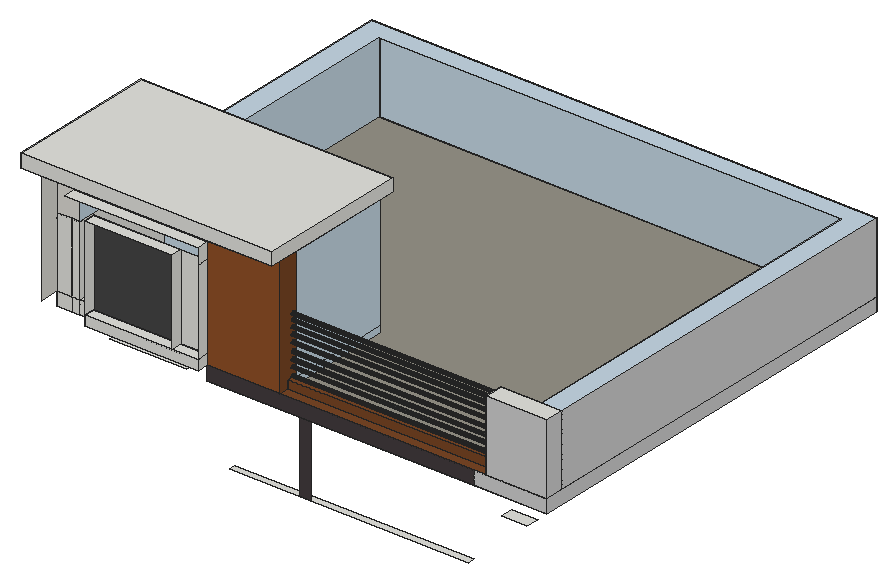
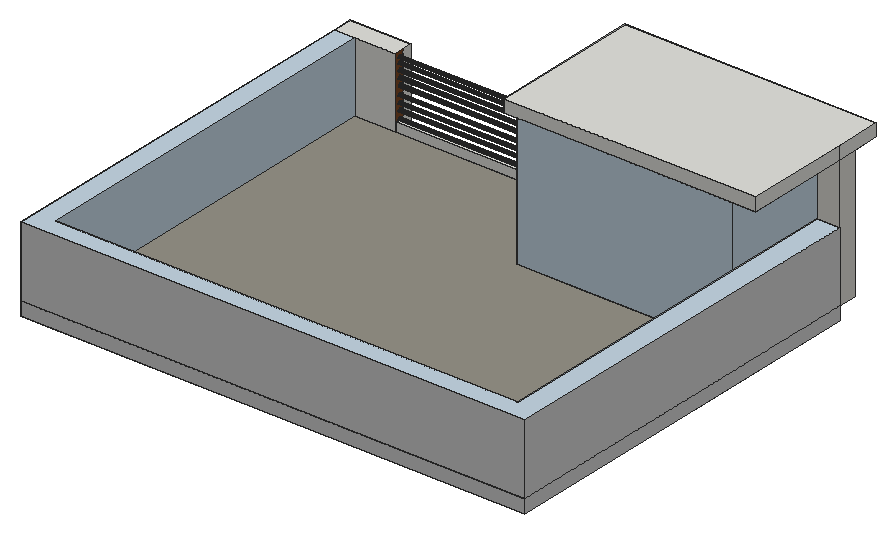
# SketchUp Ruby script. Lengths in inches.
U = 1.inch
M = Sketchup.active_model
def pt(a) = Geom::Point3d.new(a.map { |v| v * U })
def face(e, loops, mat)
  f = e.add_face(loops[0].map { |a| pt(a) })
  loops[1..].each { |l| e.add_face(l.map { |a| pt(a) }).erase! }
  f.material = f.back_material = mat if mat
  f
end
# faces: each face lists its corners as indices into pts; further lists are holes
def faces(e, pts, list, mat = nil) = list.each { |f| face(e, (f[0].is_a?(Array) ? f : [f]).map { |l| l.map { |i| pts[i] } }, mat) }
# xy, xz, yz: faces in a plane at the given z, y or x. An outline is a flat list of corners, or four numbers for a rectangle; further outlines are holes
def ring(l) = l.size == 4 ? [[l[0], l[1]], [l[2], l[1]], [l[2], l[3]], [l[0], l[3]]] : l.each_slice(2).to_a
def flat(e, list, mat, &to3) = list.each { |f| face(e, (f[0].is_a?(Array) ? f : [f]).map { |l| ring(l).map { |u, v| to3.(u, v) } }, mat) }
def xy(e, z, list, mat = nil) = flat(e, list, mat) { |x, y| [x, y, z] }
def xz(e, y, list, mat = nil) = flat(e, list, mat) { |x, z| [x, y, z] }
def yz(e, x, list, mat = nil) = flat(e, list, mat) { |y, z| [x, y, z] }
def lines(e, pts, list) = list.each { |a, b| e.add_line(pt(pts[a]), pt(pts[b])) }
# prism: a flat outline (further loops are holes) pulled along v
def prism(e, loops, v, mat = nil)
  f = face(e, loops, mat); d = Geom::Vector3d.new(v.map { |x| x * U })
  f.pushpull(f.normal.samedirection?(d) ? d.length : -d.length)
end
def box(e, o, s, mat = nil) = prism(e, [[o, [o[0] + s[0], o[1], o[2]], [o[0] + s[0], o[1] + s[1], o[2]], [o[0], o[1] + s[1], o[2]]]], [0, 0, s[2]], mat)
def at(x, y, z, deg = 0) = Geom::Transformation.translation(pt([x, y, z])) * Geom::Transformation.rotation(ORIGIN, Z_AXIS, deg.degrees)
def axes(o, x, y, z) = Geom::Transformation.new([*x, 0, *y, 0, *z, 0, *pt(o).to_a, 1])
def part(name) = M.definitions.add(name)
# library, detail: a bought-in or finely detailed component or shape, given as its bounding box
def library(name, o, s) = part(name).tap { |d| box(d.entities, o, s) }
def detail(e, o, s) = box(e.add_group.entities, o, s)
def put(e, d, t, mat = nil) = e.add_instance(d, t).tap { |i| i.material = mat if mat }
def group(e, t, mat = nil) = e.add_group.tap { |g| g.transformation = t; g.material = mat if mat }.entities
root = M.entities
M.materials.add("[Asphalt New]").color = [67, 60, 62]
M.materials.add("[Carrera Marble]").color = [207, 207, 207]
M.materials.add("[Color M07]").color = [58, 58, 58]
M.materials.add("[Formica Graystone]").color = [149, 146, 135]
M.materials.add("[Formica Laminate Dark]").color = [50, 53, 60]
M.materials.add("[Formica Laminate Light]").color = [213, 189, 164]
M.materials.add("[Granite Dark Gray]").color = [69, 68, 68]
M.materials.add("[Mirror 02]").color = [229, 229, 229]
M.materials.add("[Terrazzo Light Blue]").color = [196, 214, 227]
M.materials.add("[Terrazzo Tile Light]").color = [219, 217, 210]
M.materials.add("[Translucent Glass Gray]").color = [96, 96, 96]
M.materials["[Translucent Glass Gray]"].alpha = 0.5
M.materials.add("[Wood Cherry Original]").color = [142, 80, 39]
M.materials.add("[Wood Veneer 01]").color = [120, 70, 37]
xy(root,337.375,[[155.47,113.77,364.18,119.67]])
xy(root,386.13,[[143.73,278.02,202.85,283.21]])
xy(root,387.97,[[397.72,107.86,419.72,119.36]])
xy(root,407.4375,[[144.47,102.9,155.47,119.67],[421.41,102.9,440.93,107.86],[376,107.86,421.41,119.67],[421.41,107.86,440.93,119.67],[0,119.67,19.52,278.02],
  [421.41,119.67,440.93,278.02],[0,278.02,19.52,291.29],[19.52,278.02,378.85,291.29],[378.85,278.02,421.41,291.29],[421.41,278.02,440.93,291.29],
  [0,291.29,19.52,462.9],[19.52,291.29,365.25,443.38],[365.25,291.29,378.85,443.38],[378.85,291.29,421.41,443.38],[421.41,291.29,440.93,462.9],
  [19.52,443.38,365.25,462.9],[365.25,443.38,378.85,462.9],[378.85,443.38,421.41,462.9]])
xy(root,407.4375,[[[155.47,102.9,155.47,119.67,19.52,119.67,19.52,278.02,421.41,278.02,421.41,119.67,364.18,119.67,364.18,107.86,421.41,107.86,421.41,102.9],[216.29,107.86,226.02,113.77]]],"[Formica Laminate Light]")
xy(root,409.91,[[59.64,102.9,126.33,116.97]])
xy(root,419.375,[[45.1,93.15,144.47,102.9],[387.7,102.9,440.93,119.67],[207.97,111.29,387.7,119.67],[0,119.67,0,462.9,440.93,462.9,440.93,119.67,423.04,119.67,423.04,446.61,19.52,446.61,19.52,119.67],[19.52,119.67,144.47,211.42],
  [144.47,119.67,207.97,211.42]])
xy(root,419.375,[[207.97,119.67,423.04,119.67,423.04,446.61,19.52,446.61,19.52,211.42,207.97,211.42]],"[Formica Graystone]")
xy(root,419.375,[[207.97,102.9,387.7,111.29]],"[Wood Veneer 01]")
xy(root,426.94,[[207.97,116.04,387.7,119.67]])
xy(root,426.94,[[207.97,111.29,387.7,116.04]],"[Wood Veneer 01]")
xy(root,428.03,[[45.1,93.15,121.39,102.9],[121.39,93.15,144.47,102.9]])
xy(root,480.75,[[387.7,102.9,440.93,119.67]])
xy(root,480.75,[[0,119.67,19.52,119.67,19.52,446.61,423.04,446.61,423.04,119.67,440.93,119.67,440.93,462.9,0,462.9]],"[Terrazzo Light Blue]")
xy(root,501.96,[[45.1,93.15,121.39,102.9]])
xy(root,515.65,[[27.95,93.15,144.47,102.9]])
xy(root,533.5625,[[0,79.34,144.47,102.9],[144.47,79.34,207.97,102.9],[207.97,79.34,219.41,119.67],[0,102.9,0,119.67,19.52,119.67,19.52,211.42,207.97,211.42,207.97,102.9],[0,119.67,19.52,211.42],
  [207.97,119.67,219.41,211.42]])
xy(root,544.875,[[0,79.34,219.41,211.42]])
xz(root,79.34,[[0,533.5625,219.41,544.875]])
xz(root,93.15,[[45.1,419.375,144.47,428.03]])
xz(root,102.9,[[45.1,419.375,144.47,428.03],[121.39,428.03,144.47,501.96]])
xz(root,102.9,[[144.47,407.4375,377.08,419.375]],"[Asphalt New]")
xz(root,102.9,[[377.08,407.4375,440.93,419.375],[387.7,419.375,440.93,480.75]],"[Carrera Marble]")
xz(root,102.9,[[45.1,428.03,121.39,501.96]],"[Granite Dark Gray]")
xz(root,102.9,[[144.47,419.375,207.97,533.5625]],"[Wood Cherry Original]")
xz(root,111.29,[[207.97,419.375,387.7,426.94]],"[Wood Veneer 01]")
xz(root,113.77,[[216.29,337.375,226.02,407.4375]],"[Asphalt New]")
xz(root,119.67,[[0,407.4375,12.41,419.375],[12.41,407.4375,12.51,419.375],[12.51,407.4375,19.52,419.375],[19.52,407.4375,144.47,419.375],[0,419.375,12.41,480.75],
  [12.41,419.375,12.51,480.75],[12.51,419.375,19.52,480.75],[207.97,419.375,387.7,426.94],[387.7,419.375,423.04,480.75],[423.04,419.375,440.93,480.75]])
xz(root,119.67,[[0,480.75,19.52,533.5625]],"[Terrazzo Tile Light]")
xz(root,211.42,[[0,533.5625,219.41,544.875]])
xz(root,211.42,[[19.52,419.375,207.97,533.5625]],"[Terrazzo Light Blue]")
xz(root,278.02,[[263.57,345.67,290.95,362.74],[292.74,345.67,324.88,362.74],[263.57,365.24,290.95,384.78],[292.74,365.24,324.88,384.78]],"[Mirror 02]")
xz(root,283.21,[[170.75,329.99,173.63,383.16]],"[Formica Laminate Dark]")
xz(root,283.21,[[146.7,329.99,170.75,383.16],[173.63,329.99,199.875,383.16]],"[Translucent Glass Gray]")
xz(root,446.61,[[19.52,419.375,20.91,480.75]])
xz(root,446.61,[[20.91,419.375,423.04,480.75]],"[Terrazzo Light Blue]")
xz(root,462.9,[[0,407.4375,440.93,419.375],[0,419.375,440.93,480.75]],"[Carrera Marble]")
yz(root,0,[[79.34,533.5625,119.67,544.875],[119.67,533.5625,211.42,544.875]])
yz(root,0,[[119.67,407.4375,462.9,419.375],[119.67,419.375,462.9,480.75]],"[Carrera Marble]")
yz(root,0,[[102.9,419.375,119.67,533.5625]],"[Terrazzo Tile Light]")
yz(root,19.52,[[119.67,419.375,211.42,480.75]])
yz(root,19.52,[[211.42,419.375,446.61,480.75],[119.67,480.75,211.42,533.5625]],"[Terrazzo Light Blue]")
yz(root,45.1,[[93.15,419.375,102.9,428.03],[93.15,428.03,102.9,501.96]])
yz(root,121.39,[[93.15,428.03,102.9,501.96]])
yz(root,144.47,[[93.15,419.375,102.9,428.03],[93.15,428.03,102.9,501.96],[93.15,501.96,102.9,515.65]])
yz(root,207.97,[[111.29,419.375,119.67,426.94]])
yz(root,207.97,[[119.67,419.375,211.42,425],[119.67,425,211.42,533.5625]],"[Terrazzo Light Blue]")
yz(root,207.97,[[[102.9,419.375,111.29,419.375,111.29,426.94,119.67,426.94,119.67,533.5625,102.9,533.5625],[116.04,475.69,115.71,475.73,115.41,475.85,115.15,476.05,114.96,476.31,114.83,476.61,114.79,476.94,114.83,477.26,114.96,477.56,115.15,477.82,115.41,478.02,115.71,478.14,116.04,478.19,116.36,478.14,116.66,478.02,116.92,477.82,117.12,477.56,117.25,477.26,117.29,476.94,117.25,476.61,117.12,476.31,116.92,476.05,116.66,475.85,116.36,475.73],[116.04,470.81,115.71,470.85,115.41,470.98,115.15,471.18,114.96,471.44,114.83,471.74,114.79,472.06,114.83,472.38,114.96,472.69,115.15,472.94,115.41,473.14,115.71,473.27,116.04,473.31,116.36,473.27,116.66,473.14,116.92,472.94,117.12,472.69,117.25,472.38,117.29,472.06,117.25,471.74,117.12,471.44,116.92,471.18,116.66,470.98,116.36,470.85],[116.04,465.19,115.71,465.23,115.41,465.35,115.15,465.55,114.96,465.81,114.83,466.11,114.79,466.44,114.83,466.76,114.96,467.06,115.15,467.32,115.41,467.52,115.71,467.64,116.04,467.69,116.36,467.64,116.66,467.52,116.92,467.32,117.12,467.06,117.25,466.76,117.29,466.44,117.25,466.11,117.12,465.81,116.92,465.55,116.66,465.35,116.36,465.23],[116.04,459.44,115.71,459.48,115.41,459.6,115.15,459.8,114.96,460.06,114.83,460.36,114.79,460.69,114.83,461.01,114.96,461.31,115.15,461.57,115.41,461.77,115.71,461.89,116.04,461.94,116.36,461.89,116.66,461.77,116.92,461.57,117.12,461.31,117.25,461.01,117.29,460.69,117.25,460.36,117.12,460.06,116.92,459.8,116.66,459.6,116.36,459.48],[116.04,453.19,115.71,453.23,115.41,453.35,115.15,453.55,114.96,453.81,114.83,454.11,114.79,454.44,114.83,454.76,114.96,455.06,115.15,455.32,115.41,455.52,115.71,455.64,116.04,455.69,116.36,455.64,116.66,455.52,116.92,455.32,117.12,455.06,117.25,454.76,117.29,454.44,117.25,454.11,117.12,453.81,116.92,453.55,116.66,453.35,116.36,453.23],[116.04,446,115.71,446.04,115.41,446.17,115.15,446.36,114.96,446.62,114.83,446.92,114.79,447.25,114.83,447.57,114.96,447.87,115.15,448.13,115.41,448.33,115.71,448.45,116.04,448.5,116.36,448.45,116.66,448.33,116.92,448.13,117.12,447.87,117.25,447.57,117.29,447.25,117.25,446.92,117.12,446.62,116.92,446.36,116.66,446.17,116.36,446.04],[116.04,426.94,115.71,426.98,115.41,427.1,115.15,427.3,114.96,427.56,114.83,427.86,114.79,428.19,114.83,428.51,114.96,428.81,115.15,429.07,115.41,429.27,115.71,429.39,116.04,429.44,116.36,429.39,116.66,429.27,116.92,429.07,117.12,428.81,117.25,428.51,117.29,428.19,117.25,427.86,117.12,427.56,116.92,427.3,116.66,427.1,116.36,426.98],[116.04,433.87,115.71,433.92,115.41,434.04,115.15,434.24,114.96,434.5,114.83,434.8,114.79,435.12,114.83,435.45,114.96,435.75,115.15,436.01,115.41,436.21,115.71,436.33,116.04,436.37,116.36,436.33,116.66,436.21,116.92,436.01,117.12,435.75,117.25,435.45,117.29,435.12,117.25,434.8,117.12,434.5,116.92,434.24,116.66,434.04,116.36,433.92],[116.04,439.69,115.71,439.73,115.41,439.85,115.15,440.05,114.96,440.31,114.83,440.61,114.79,440.94,114.83,441.26,114.96,441.56,115.15,441.82,115.41,442.02,115.71,442.14,116.04,442.19,116.36,442.14,116.66,442.02,116.92,441.82,117.12,441.56,117.25,441.26,117.29,440.94,117.25,440.61,117.12,440.31,116.92,440.05,116.66,439.85,116.36,439.73]]],"[Wood Veneer 01]")
yz(root,219.41,[[79.34,533.5625,211.42,544.875]])
yz(root,387.7,[[102.9,419.375,111.29,480.75],[111.29,419.375,119.67,426.94],[116.04,426.94,116.36,426.98,116.66,427.1,116.92,427.3,117.12,427.56,117.25,427.86,117.29,428.19,117.25,428.51,117.12,428.81,116.92,429.07,116.66,429.27,116.36,429.39,116.04,429.44,115.71,429.39,115.41,429.27,115.15,429.07,114.96,428.81,114.83,428.51,114.79,428.19,114.83,427.86,114.96,427.56,115.15,427.3,115.41,427.1,115.71,426.98],[116.04,433.87,116.36,433.92,116.66,434.04,116.92,434.24,117.12,434.5,117.25,434.8,117.29,435.12,117.25,435.45,117.12,435.75,116.92,436.01,116.66,436.21,116.36,436.33,116.04,436.37,115.71,436.33,115.41,436.21,115.15,436.01,114.96,435.75,114.83,435.45,114.79,435.12,114.83,434.8,114.96,434.5,115.15,434.24,115.41,434.04,115.71,433.92],[116.04,439.69,116.36,439.73,116.66,439.85,116.92,440.05,117.12,440.31,117.25,440.61,117.29,440.94,117.25,441.26,117.12,441.56,116.92,441.82,116.66,442.02,116.36,442.14,116.04,442.19,115.71,442.14,115.41,442.02,115.15,441.82,114.96,441.56,114.83,441.26,114.79,440.94,114.83,440.61,114.96,440.31,115.15,440.05,115.41,439.85,115.71,439.73],
  [116.04,446,116.36,446.04,116.66,446.17,116.92,446.36,117.12,446.62,117.25,446.92,117.29,447.25,117.25,447.57,117.12,447.87,116.92,448.13,116.66,448.33,116.36,448.45,116.04,448.5,115.71,448.45,115.41,448.33,115.15,448.13,114.96,447.87,114.83,447.57,114.79,447.25,114.83,446.92,114.96,446.62,115.15,446.36,115.41,446.17,115.71,446.04],[116.04,453.19,116.36,453.23,116.66,453.35,116.92,453.55,117.12,453.81,117.25,454.11,117.29,454.44,117.25,454.76,117.12,455.06,116.92,455.32,116.66,455.52,116.36,455.64,116.04,455.69,115.71,455.64,115.41,455.52,115.15,455.32,114.96,455.06,114.83,454.76,114.79,454.44,114.83,454.11,114.96,453.81,115.15,453.55,115.41,453.35,115.71,453.23],[116.04,459.44,116.36,459.48,116.66,459.6,116.92,459.8,117.12,460.06,117.25,460.36,117.29,460.69,117.25,461.01,117.12,461.31,116.92,461.57,116.66,461.77,116.36,461.89,116.04,461.94,115.71,461.89,115.41,461.77,115.15,461.57,114.96,461.31,114.83,461.01,114.79,460.69,114.83,460.36,114.96,460.06,115.15,459.8,115.41,459.6,115.71,459.48],[116.04,465.19,116.36,465.23,116.66,465.35,116.92,465.55,117.12,465.81,117.25,466.11,117.29,466.44,117.25,466.76,117.12,467.06,116.92,467.32,116.66,467.52,116.36,467.64,116.04,467.69,115.71,467.64,115.41,467.52,115.15,467.32,114.96,467.06,114.83,466.76,114.79,466.44,114.83,466.11,114.96,465.81,115.15,465.55,115.41,465.35,115.71,465.23],[116.04,470.81,116.36,470.85,116.66,470.98,116.92,471.18,117.12,471.44,117.25,471.74,117.29,472.06,117.25,472.38,117.12,472.69,116.92,472.94,116.66,473.14,116.36,473.27,116.04,473.31,115.71,473.27,115.41,473.14,115.15,472.94,114.96,472.69,114.83,472.38,114.79,472.06,114.83,471.74,114.96,471.44,115.15,471.18,115.41,470.98,115.71,470.85],
  [116.04,475.69,116.36,475.73,116.66,475.85,116.92,476.05,117.12,476.31,117.25,476.61,117.29,476.94,117.25,477.26,117.12,477.56,116.92,477.82,116.66,478.02,116.36,478.14,116.04,478.19,115.71,478.14,115.41,478.02,115.15,477.82,114.96,477.56,114.83,477.26,114.79,476.94,114.83,476.61,114.96,476.31,115.15,476.05,115.41,475.85,115.71,475.73]])
yz(root,387.7,[[[111.29,426.94,119.67,480.75],[116.04,475.69,116.36,475.73,116.66,475.85,116.92,476.05,117.12,476.31,117.25,476.61,117.29,476.94,117.25,477.26,117.12,477.56,116.92,477.82,116.66,478.02,116.36,478.14,116.04,478.19,115.71,478.14,115.41,478.02,115.15,477.82,114.96,477.56,114.83,477.26,114.79,476.94,114.83,476.61,114.96,476.31,115.15,476.05,115.41,475.85,115.71,475.73],[116.04,426.94,116.36,426.98,116.66,427.1,116.92,427.3,117.12,427.56,117.25,427.86,117.29,428.19,117.25,428.51,117.12,428.81,116.92,429.07,116.66,429.27,116.36,429.39,116.04,429.44,115.71,429.39,115.41,429.27,115.15,429.07,114.96,428.81,114.83,428.51,114.79,428.19,114.83,427.86,114.96,427.56,115.15,427.3,115.41,427.1,115.71,426.98],[116.04,470.81,116.36,470.85,116.66,470.98,116.92,471.18,117.12,471.44,117.25,471.74,117.29,472.06,117.25,472.38,117.12,472.69,116.92,472.94,116.66,473.14,116.36,473.27,116.04,473.31,115.71,473.27,115.41,473.14,115.15,472.94,114.96,472.69,114.83,472.38,114.79,472.06,114.83,471.74,114.96,471.44,115.15,471.18,115.41,470.98,115.71,470.85],[116.04,433.87,116.36,433.92,116.66,434.04,116.92,434.24,117.12,434.5,117.25,434.8,117.29,435.12,117.25,435.45,117.12,435.75,116.92,436.01,116.66,436.21,116.36,436.33,116.04,436.37,115.71,436.33,115.41,436.21,115.15,436.01,114.96,435.75,114.83,435.45,114.79,435.12,114.83,434.8,114.96,434.5,115.15,434.24,115.41,434.04,115.71,433.92],[116.04,465.19,116.36,465.23,116.66,465.35,116.92,465.55,117.12,465.81,117.25,466.11,117.29,466.44,117.25,466.76,117.12,467.06,116.92,467.32,116.66,467.52,116.36,467.64,116.04,467.69,115.71,467.64,115.41,467.52,115.15,467.32,114.96,467.06,114.83,466.76,114.79,466.44,114.83,466.11,114.96,465.81,115.15,465.55,115.41,465.35,115.71,465.23],[116.04,439.69,116.36,439.73,116.66,439.85,116.92,440.05,117.12,440.31,117.25,440.61,117.29,440.94,117.25,441.26,117.12,441.56,116.92,441.82,116.66,442.02,116.36,442.14,116.04,442.19,115.71,442.14,115.41,442.02,115.15,441.82,114.96,441.56,114.83,441.26,114.79,440.94,114.83,440.61,114.96,440.31,115.15,440.05,115.41,439.85,115.71,439.73],[116.04,459.44,116.36,459.48,116.66,459.6,116.92,459.8,117.12,460.06,117.25,460.36,117.29,460.69,117.25,461.01,117.12,461.31,116.92,461.57,116.66,461.77,116.36,461.89,116.04,461.94,115.71,461.89,115.41,461.77,115.15,461.57,114.96,461.31,114.83,461.01,114.79,460.69,114.83,460.36,114.96,460.06,115.15,459.8,115.41,459.6,115.71,459.48],[116.04,446,116.36,446.04,116.66,446.17,116.92,446.36,117.12,446.62,117.25,446.92,117.29,447.25,117.25,447.57,117.12,447.87,116.92,448.13,116.66,448.33,116.36,448.45,116.04,448.5,115.71,448.45,115.41,448.33,115.15,448.13,114.96,447.87,114.83,447.57,114.79,447.25,114.83,446.92,114.96,446.62,115.15,446.36,115.41,446.17,115.71,446.04],[116.04,453.19,116.36,453.23,116.66,453.35,116.92,453.55,117.12,453.81,117.25,454.11,117.29,454.44,117.25,454.76,117.12,455.06,116.92,455.32,116.66,455.52,116.36,455.64,116.04,455.69,115.71,455.64,115.41,455.52,115.15,455.32,114.96,455.06,114.83,454.76,114.79,454.44,114.83,454.11,114.96,453.81,115.15,453.55,115.41,453.35,115.71,453.23]]],"[Wood Veneer 01]")
yz(root,423.04,[[119.67,419.375,446.61,480.75]],"[Terrazzo Light Blue]")
yz(root,440.93,[[102.9,407.4375,462.9,419.375],[102.9,419.375,119.67,480.75],[119.67,419.375,462.9,480.75]],"[Carrera Marble]")
p = [[387.7,116.04,426.94],[387.7,115.71,426.98],[207.97,115.71,426.98],[207.97,116.04,426.94],[387.7,116.36,426.98],[207.97,116.36,426.98],
  [387.7,115.41,427.1],[207.97,115.41,427.1],[387.7,116.66,427.1],[207.97,116.66,427.1],[387.7,115.15,427.3],[207.97,115.15,427.3],
  [387.7,116.92,427.3],[207.97,116.92,427.3],[387.7,114.96,427.56],[207.97,114.96,427.56],[387.7,117.12,427.56],[207.97,117.12,427.56],
  [387.7,114.83,427.86],[207.97,114.83,427.86],[387.7,117.25,427.86],[207.97,117.25,427.86],[387.7,114.79,428.19],[207.97,114.79,428.19],
  [387.7,117.29,428.19],[207.97,117.29,428.19],[387.7,114.83,428.51],[207.97,114.83,428.51],[387.7,117.25,428.51],[207.97,117.25,428.51],
  [387.7,114.96,428.81],[207.97,114.96,428.81],[387.7,117.12,428.81],[207.97,117.12,428.81],[387.7,115.15,429.07],[207.97,115.15,429.07],
  [387.7,116.92,429.07],[207.97,116.92,429.07],[387.7,115.41,429.27],[207.97,115.41,429.27],[387.7,116.66,429.27],[207.97,116.66,429.27],
  [387.7,115.71,429.39],[207.97,115.71,429.39],[387.7,116.36,429.39],[207.97,116.36,429.39],[387.7,116.04,429.44],[207.97,116.04,429.44],
  [387.7,115.71,433.92],[387.7,115.41,434.04],[207.97,115.41,434.04],[207.97,115.71,433.92],[387.7,116.04,433.87],[207.97,116.04,433.87],
  [387.7,116.36,433.92],[207.97,116.36,433.92],[387.7,116.66,434.04],[207.97,116.66,434.04],[387.7,115.15,434.24],[207.97,115.15,434.24],
  [387.7,116.92,434.24],[207.97,116.92,434.24],[387.7,114.96,434.5],[207.97,114.96,434.5],[387.7,117.12,434.5],[207.97,117.12,434.5],
  [387.7,114.83,434.8],[207.97,114.83,434.8],[387.7,117.25,434.8],[207.97,117.25,434.8],[387.7,114.79,435.12],[207.97,114.79,435.12],
  [387.7,117.29,435.12],[207.97,117.29,435.12],[387.7,114.83,435.45],[207.97,114.83,435.45],[387.7,117.25,435.45],[207.97,117.25,435.45],
  [387.7,114.96,435.75],[207.97,114.96,435.75],[387.7,117.12,435.75],[207.97,117.12,435.75],[387.7,115.15,436.01],[207.97,115.15,436.01],
  [387.7,116.92,436.01],[207.97,116.92,436.01],[387.7,115.41,436.21],[207.97,115.41,436.21],[387.7,116.66,436.21],[207.97,116.66,436.21],
  [387.7,115.71,436.33],[207.97,115.71,436.33],[387.7,116.36,436.33],[207.97,116.36,436.33],[387.7,116.04,436.37],[207.97,116.04,436.37],
  [387.7,115.71,439.73],[387.7,115.41,439.85],[207.97,115.41,439.85],[207.97,115.71,439.73],[387.7,116.04,439.69],[207.97,116.04,439.69],
  [387.7,116.36,439.73],[207.97,116.36,439.73],[387.7,116.66,439.85],[207.97,116.66,439.85],[387.7,115.15,440.05],[207.97,115.15,440.05],
  [387.7,116.92,440.05],[207.97,116.92,440.05],[387.7,114.96,440.31],[207.97,114.96,440.31],[387.7,117.12,440.31],[207.97,117.12,440.31],
  [387.7,114.83,440.61],[207.97,114.83,440.61],[387.7,117.25,440.61],[207.97,117.25,440.61],[387.7,114.79,440.94],[207.97,114.79,440.94],
  [387.7,117.29,440.94],[207.97,117.29,440.94],[387.7,114.83,441.26],[207.97,114.83,441.26],[387.7,117.25,441.26],[207.97,117.25,441.26],
  [387.7,114.96,441.56],[207.97,114.96,441.56],[387.7,117.12,441.56],[207.97,117.12,441.56],[387.7,115.15,441.82],[207.97,115.15,441.82],
  [387.7,116.92,441.82],[207.97,116.92,441.82],[387.7,115.41,442.02],[207.97,115.41,442.02],[387.7,116.66,442.02],[207.97,116.66,442.02],
  [387.7,115.71,442.14],[207.97,115.71,442.14],[387.7,116.36,442.14],[207.97,116.36,442.14],[387.7,116.04,442.19],[207.97,116.04,442.19],
  [387.7,115.71,446.04],[387.7,115.41,446.17],[207.97,115.41,446.17],[207.97,115.71,446.04],[387.7,116.04,446],[207.97,116.04,446],
  [387.7,116.36,446.04],[207.97,116.36,446.04],[387.7,116.66,446.17],[207.97,116.66,446.17],[387.7,115.15,446.36],[207.97,115.15,446.36],
  [387.7,116.92,446.36],[207.97,116.92,446.36],[387.7,114.96,446.62],[207.97,114.96,446.62],[387.7,117.12,446.62],[207.97,117.12,446.62],
  [387.7,114.83,446.92],[207.97,114.83,446.92],[387.7,117.25,446.92],[207.97,117.25,446.92],[387.7,114.79,447.25],[207.97,114.79,447.25],
  [387.7,117.29,447.25],[207.97,117.29,447.25],[387.7,114.83,447.57],[207.97,114.83,447.57],[387.7,117.25,447.57],[207.97,117.25,447.57],
  [387.7,114.96,447.87],[207.97,114.96,447.87],[387.7,117.12,447.87],[207.97,117.12,447.87],[387.7,115.15,448.13],[207.97,115.15,448.13],
  [387.7,116.92,448.13],[207.97,116.92,448.13],[387.7,115.41,448.33],[207.97,115.41,448.33],[387.7,116.66,448.33],[207.97,116.66,448.33],
  [387.7,115.71,448.45],[207.97,115.71,448.45],[387.7,116.36,448.45],[207.97,116.36,448.45],[387.7,116.04,448.5],[207.97,116.04,448.5],
  [387.7,115.71,453.23],[387.7,115.41,453.35],[207.97,115.41,453.35],[207.97,115.71,453.23],[387.7,116.04,453.19],[207.97,116.04,453.19],
  [387.7,116.36,453.23],[207.97,116.36,453.23],[387.7,116.66,453.35],[207.97,116.66,453.35],[387.7,115.15,453.55],[207.97,115.15,453.55],
  [387.7,116.92,453.55],[207.97,116.92,453.55],[387.7,114.96,453.81],[207.97,114.96,453.81],[387.7,117.12,453.81],[207.97,117.12,453.81],
  [387.7,114.83,454.11],[207.97,114.83,454.11],[387.7,117.25,454.11],[207.97,117.25,454.11],[387.7,114.79,454.44],[207.97,114.79,454.44],
  [387.7,117.29,454.44],[207.97,117.29,454.44],[387.7,114.83,454.76],[207.97,114.83,454.76],[387.7,117.25,454.76],[207.97,117.25,454.76],
  [387.7,114.96,455.06],[207.97,114.96,455.06],[387.7,117.12,455.06],[207.97,117.12,455.06],[387.7,115.15,455.32],[207.97,115.15,455.32],
  [387.7,116.92,455.32],[207.97,116.92,455.32],[387.7,115.41,455.52],[207.97,115.41,455.52],[387.7,116.66,455.52],[207.97,116.66,455.52],
  [387.7,115.71,455.64],[207.97,115.71,455.64],[387.7,116.36,455.64],[207.97,116.36,455.64],[387.7,116.04,455.69],[207.97,116.04,455.69],
  [387.7,116.04,459.44],[387.7,115.71,459.48],[207.97,115.71,459.48],[207.97,116.04,459.44],[387.7,116.36,459.48],[207.97,116.36,459.48],
  [387.7,115.41,459.6],[207.97,115.41,459.6],[387.7,116.66,459.6],[207.97,116.66,459.6],[387.7,115.15,459.8],[207.97,115.15,459.8],
  [387.7,116.92,459.8],[207.97,116.92,459.8],[387.7,114.96,460.06],[207.97,114.96,460.06],[387.7,117.12,460.06],[207.97,117.12,460.06],
  [387.7,114.83,460.36],[207.97,114.83,460.36],[387.7,117.25,460.36],[207.97,117.25,460.36],[387.7,114.79,460.69],[207.97,114.79,460.69],
  [387.7,117.29,460.69],[207.97,117.29,460.69],[387.7,114.83,461.01],[207.97,114.83,461.01],[387.7,117.25,461.01],[207.97,117.25,461.01],
  [387.7,114.96,461.31],[207.97,114.96,461.31],[387.7,117.12,461.31],[207.97,117.12,461.31],[387.7,115.15,461.57],[207.97,115.15,461.57],
  [387.7,116.92,461.57],[207.97,116.92,461.57],[387.7,115.41,461.77],[207.97,115.41,461.77],[387.7,116.66,461.77],[207.97,116.66,461.77],
  [387.7,115.71,461.89],[207.97,115.71,461.89],[387.7,116.36,461.89],[207.97,116.36,461.89],[387.7,116.04,461.94],[207.97,116.04,461.94],
  [387.7,115.71,465.23],[387.7,115.41,465.35],[207.97,115.41,465.35],[207.97,115.71,465.23],[387.7,116.04,465.19],[207.97,116.04,465.19],
  [387.7,116.36,465.23],[207.97,116.36,465.23],[387.7,116.66,465.35],[207.97,116.66,465.35],[387.7,115.15,465.55],[207.97,115.15,465.55],
  [387.7,116.92,465.55],[207.97,116.92,465.55],[387.7,114.96,465.81],[207.97,114.96,465.81],[387.7,117.12,465.81],[207.97,117.12,465.81],
  [387.7,114.83,466.11],[207.97,114.83,466.11],[387.7,117.25,466.11],[207.97,117.25,466.11],[387.7,114.79,466.44],[207.97,114.79,466.44],
  [387.7,117.29,466.44],[207.97,117.29,466.44],[387.7,114.83,466.76],[207.97,114.83,466.76],[387.7,117.25,466.76],[207.97,117.25,466.76],
  [387.7,114.96,467.06],[207.97,114.96,467.06],[387.7,117.12,467.06],[207.97,117.12,467.06],[387.7,115.15,467.32],[207.97,115.15,467.32],
  [387.7,116.92,467.32],[207.97,116.92,467.32],[387.7,115.41,467.52],[207.97,115.41,467.52],[387.7,116.66,467.52],[207.97,116.66,467.52],
  [387.7,115.71,467.64],[207.97,115.71,467.64],[387.7,116.36,467.64],[207.97,116.36,467.64],[387.7,116.04,467.69],[207.97,116.04,467.69],
  [387.7,116.04,470.81],[387.7,115.71,470.85],[207.97,115.71,470.85],[207.97,116.04,470.81],[387.7,116.36,470.85],[207.97,116.36,470.85],
  [387.7,115.41,470.98],[207.97,115.41,470.98],[387.7,116.66,470.98],[207.97,116.66,470.98],[387.7,115.15,471.18],[207.97,115.15,471.18],
  [387.7,116.92,471.18],[207.97,116.92,471.18],[387.7,114.96,471.44],[207.97,114.96,471.44],[387.7,117.12,471.44],[207.97,117.12,471.44],
  [387.7,114.83,471.74],[207.97,114.83,471.74],[387.7,117.25,471.74],[207.97,117.25,471.74],[387.7,114.79,472.06],[207.97,114.79,472.06],
  [387.7,117.29,472.06],[207.97,117.29,472.06],[387.7,114.83,472.38],[207.97,114.83,472.38],[387.7,117.25,472.38],[207.97,117.25,472.38],
  [387.7,114.96,472.69],[207.97,114.96,472.69],[387.7,117.12,472.69],[207.97,117.12,472.69],[387.7,115.15,472.94],[207.97,115.15,472.94],
  [387.7,116.92,472.94],[207.97,116.92,472.94],[387.7,115.41,473.14],[207.97,115.41,473.14],[387.7,116.66,473.14],[207.97,116.66,473.14],
  [387.7,115.71,473.27],[207.97,115.71,473.27],[387.7,116.36,473.27],[207.97,116.36,473.27],[387.7,116.04,473.31],[207.97,116.04,473.31],
  [387.7,115.71,475.73],[387.7,115.41,475.85],[207.97,115.41,475.85],[207.97,115.71,475.73],[387.7,116.04,475.69],[207.97,116.04,475.69],
  [387.7,116.36,475.73],[207.97,116.36,475.73],[387.7,116.66,475.85],[207.97,116.66,475.85],[387.7,115.15,476.05],[207.97,115.15,476.05],
  [387.7,116.92,476.05],[207.97,116.92,476.05],[387.7,114.96,476.31],[207.97,114.96,476.31],[387.7,117.12,476.31],[207.97,117.12,476.31],
  [387.7,114.83,476.61],[207.97,114.83,476.61],[387.7,117.25,476.61],[207.97,117.25,476.61],[387.7,114.79,476.94],[207.97,114.79,476.94],
  [387.7,117.29,476.94],[207.97,117.29,476.94],[387.7,114.83,477.26],[207.97,114.83,477.26],[387.7,117.25,477.26],[207.97,117.25,477.26],
  [387.7,114.96,477.56],[207.97,114.96,477.56],[387.7,117.12,477.56],[207.97,117.12,477.56],[387.7,115.15,477.82],[207.97,115.15,477.82],
  [387.7,116.92,477.82],[207.97,116.92,477.82],[387.7,115.41,478.02],[207.97,115.41,478.02],[387.7,116.66,478.02],[207.97,116.66,478.02],
  [387.7,115.71,478.14],[207.97,115.71,478.14],[387.7,116.36,478.14],[207.97,116.36,478.14],[387.7,116.04,478.19],[207.97,116.04,478.19]]
faces(root,p,[[0,1,2,3],[4,0,3,5],[1,6,7,2],[8,4,5,9],[6,10,11,7],[12,8,9,13],[10,14,15,11],[16,12,13,17],
  [14,18,19,15],[20,16,17,21],[18,22,23,19],[24,20,21,25],[22,26,27,23],[28,24,25,29],[26,30,31,27],[32,28,29,33],
  [30,34,35,31],[36,32,33,37],[34,38,39,35],[40,36,37,41],[38,42,43,39],[44,40,41,45],[42,46,47,43],[46,44,45,47],
  [48,49,50,51],[52,48,51,53],[54,52,53,55],[56,54,55,57],[49,58,59,50],[60,56,57,61],[58,62,63,59],[64,60,61,65],
  [62,66,67,63],[68,64,65,69],[66,70,71,67],[72,68,69,73],[70,74,75,71],[76,72,73,77],[74,78,79,75],[80,76,77,81],
  [78,82,83,79],[84,80,81,85],[82,86,87,83],[88,84,85,89],[86,90,91,87],[92,88,89,93],[90,94,95,91],[94,92,93,95],
  [96,97,98,99],[100,96,99,101],[102,100,101,103],[104,102,103,105],[97,106,107,98],[108,104,105,109],[106,110,111,107],[112,108,109,113],
  [110,114,115,111],[116,112,113,117],[114,118,119,115],[120,116,117,121],[118,122,123,119],[124,120,121,125],[122,126,127,123],[128,124,125,129],
  [126,130,131,127],[132,128,129,133],[130,134,135,131],[136,132,133,137],[134,138,139,135],[140,136,137,141],[138,142,143,139],[142,140,141,143],
  [144,145,146,147],[148,144,147,149],[150,148,149,151],[152,150,151,153],[145,154,155,146],[156,152,153,157],[154,158,159,155],[160,156,157,161],
  [158,162,163,159],[164,160,161,165],[162,166,167,163],[168,164,165,169],[166,170,171,167],[172,168,169,173],[170,174,175,171],[176,172,173,177],
  [174,178,179,175],[180,176,177,181],[178,182,183,179],[184,180,181,185],[182,186,187,183],[188,184,185,189],[186,190,191,187],[190,188,189,191],
  [192,193,194,195],[196,192,195,197],[198,196,197,199],[200,198,199,201],[193,202,203,194],[204,200,201,205],[202,206,207,203],[208,204,205,209],
  [206,210,211,207],[212,208,209,213],[210,214,215,211],[216,212,213,217],[214,218,219,215],[220,216,217,221],[218,222,223,219],[224,220,221,225],
  [222,226,227,223],[228,224,225,229],[226,230,231,227],[232,228,229,233],[230,234,235,231],[236,232,233,237],[234,238,239,235],[238,236,237,239],
  [240,241,242,243],[244,240,243,245],[241,246,247,242],[248,244,245,249],[246,250,251,247],[252,248,249,253],[250,254,255,251],[256,252,253,257],
  [254,258,259,255],[260,256,257,261],[258,262,263,259],[264,260,261,265],[262,266,267,263],[268,264,265,269],[266,270,271,267],[272,268,269,273],
  [270,274,275,271],[276,272,273,277],[274,278,279,275],[280,276,277,281],[278,282,283,279],[284,280,281,285],[282,286,287,283],[286,284,285,287],
  [288,289,290,291],[292,288,291,293],[294,292,293,295],[296,294,295,297],[289,298,299,290],[300,296,297,301],[298,302,303,299],[304,300,301,305],
  [302,306,307,303],[308,304,305,309],[306,310,311,307],[312,308,309,313],[310,314,315,311],[316,312,313,317],[314,318,319,315],[320,316,317,321],
  [318,322,323,319],[324,320,321,325],[322,326,327,323],[328,324,325,329],[326,330,331,327],[332,328,329,333],[330,334,335,331],[334,332,333,335],
  [336,337,338,339],[340,336,339,341],[337,342,343,338],[344,340,341,345],[342,346,347,343],[348,344,345,349],[346,350,351,347],[352,348,349,353],
  [350,354,355,351],[356,352,353,357],[354,358,359,355],[360,356,357,361],[358,362,363,359],[364,360,361,365],[362,366,367,363],[368,364,365,369],
  [366,370,371,367],[372,368,369,373],[370,374,375,371],[376,372,373,377],[374,378,379,375],[380,376,377,381],[378,382,383,379],[382,380,381,383],
  [384,385,386,387],[388,384,387,389],[390,388,389,391],[392,390,391,393],[385,394,395,386],[396,392,393,397],[394,398,399,395],[400,396,397,401],
  [398,402,403,399],[404,400,401,405],[402,406,407,403],[408,404,405,409],[406,410,411,407],[412,408,409,413],[410,414,415,411],[416,412,413,417],
  [414,418,419,415],[420,416,417,421],[418,422,423,419],[424,420,421,425],[422,426,427,423],[428,424,425,429],[426,430,431,427],[430,428,429,431]],"[Color M07]")
